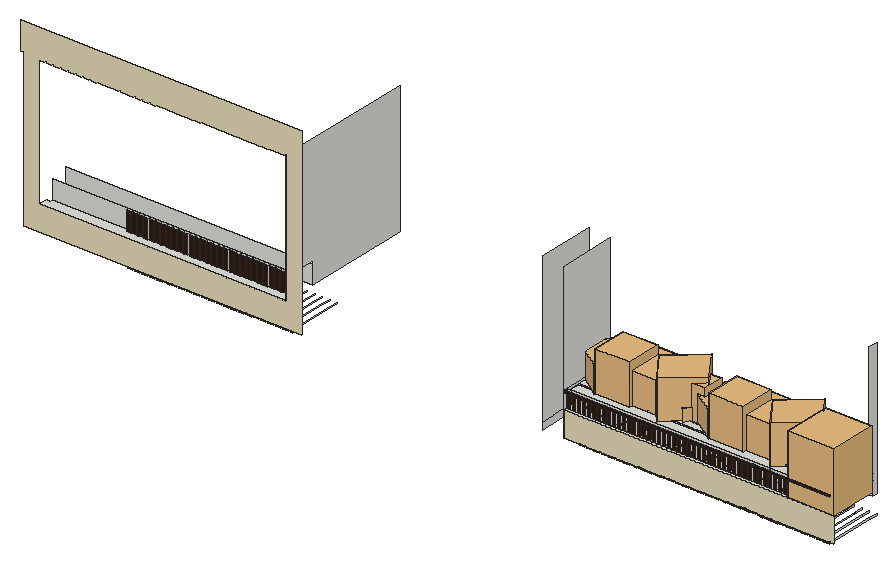
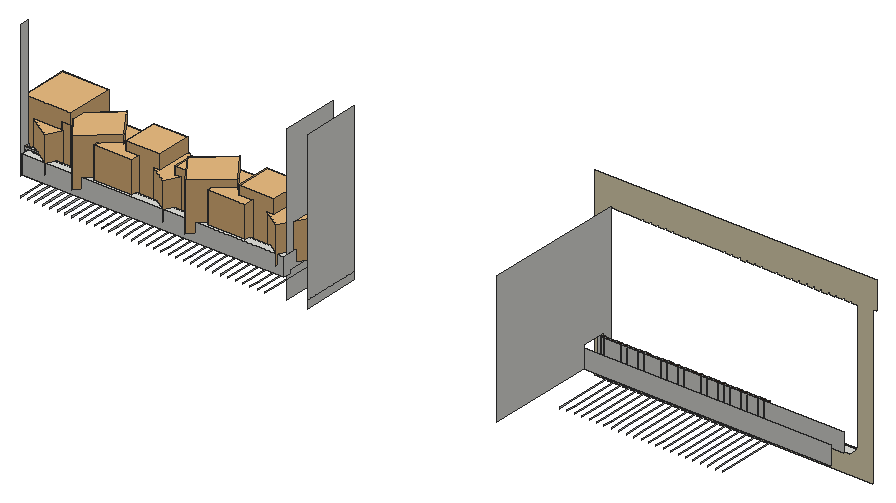
# SketchUp Ruby script. Lengths in inches.
U = 1.inch
M = Sketchup.active_model
def pt(a) = Geom::Point3d.new(a.map { |v| v * U })
def face(e, loops, mat)
  f = e.add_face(loops[0].map { |a| pt(a) })
  loops[1..].each { |l| e.add_face(l.map { |a| pt(a) }).erase! }
  f.material = f.back_material = mat if mat
  f
end
# faces: each face lists its corners as indices into pts; further lists are holes
def faces(e, pts, list, mat = nil) = list.each { |f| face(e, (f[0].is_a?(Array) ? f : [f]).map { |l| l.map { |i| pts[i] } }, mat) }
# xy, xz, yz: faces in a plane at the given z, y or x. An outline is a flat list of corners, or four numbers for a rectangle; further outlines are holes
def ring(l) = l.size == 4 ? [[l[0], l[1]], [l[2], l[1]], [l[2], l[3]], [l[0], l[3]]] : l.each_slice(2).to_a
def flat(e, list, mat, &to3) = list.each { |f| face(e, (f[0].is_a?(Array) ? f : [f]).map { |l| ring(l).map { |u, v| to3.(u, v) } }, mat) }
def xy(e, z, list, mat = nil) = flat(e, list, mat) { |x, y| [x, y, z] }
def xz(e, y, list, mat = nil) = flat(e, list, mat) { |x, z| [x, y, z] }
def yz(e, x, list, mat = nil) = flat(e, list, mat) { |y, z| [x, y, z] }
def lines(e, pts, list) = list.each { |a, b| e.add_line(pt(pts[a]), pt(pts[b])) }
# prism: a flat outline (further loops are holes) pulled along v
def prism(e, loops, v, mat = nil)
  f = face(e, loops, mat); d = Geom::Vector3d.new(v.map { |x| x * U })
  f.pushpull(f.normal.samedirection?(d) ? d.length : -d.length)
end
def box(e, o, s, mat = nil) = prism(e, [[o, [o[0] + s[0], o[1], o[2]], [o[0] + s[0], o[1] + s[1], o[2]], [o[0], o[1] + s[1], o[2]]]], [0, 0, s[2]], mat)
def at(x, y, z, deg = 0) = Geom::Transformation.translation(pt([x, y, z])) * Geom::Transformation.rotation(ORIGIN, Z_AXIS, deg.degrees)
def axes(o, x, y, z) = Geom::Transformation.new([*x, 0, *y, 0, *z, 0, *pt(o).to_a, 1])
def part(name) = M.definitions.add(name)
# library, detail: a bought-in or finely detailed component or shape, given as its bounding box
def library(name, o, s) = part(name).tap { |d| box(d.entities, o, s) }
def detail(e, o, s) = box(e.add_group.entities, o, s)
def put(e, d, t, mat = nil) = e.add_instance(d, t).tap { |i| i.material = mat if mat }
def group(e, t, mat = nil) = e.add_group.tap { |g| g.transformation = t; g.material = mat if mat }.entities
root = M.entities
M.materials.add("Material__1").color = [95, 70, 46]
M.materials.add("[Color D01]").color = [237, 225, 189]
M.materials.add("[Wood Veneer 01]").color = [51, 28, 15]
c1 = library("Areca palm plant",[0,0,0],[49.1,36.6,54.46])
c2 = library("Group\#74",[-84.69,-90.07,-0.36],[176.51,175.13,171.4])
c3 = library("Group20\#1",[-20.81,-17.08,3.79],[39.86,39.43,37.51])
c4 = library("Group\#130",[-7.34,-1.2,0],[38.67,35.81,49.04])
c5 = library("Group38\#2",[14.01,28.44,-23.43],[18.58,18.32,38.89])
c6 = part("Group\#16")
put(c6.entities,c1,axes([-6.2,158.41,6.08],[0.45017,-0.56191,0],[0.66137,0.52986,0],[0,0,0.72]))
put(c6.entities,c1,axes([-6.2,56.6,6.08],[0.45017,-0.56191,0],[0.66137,0.52986,0],[0,0,0.72]))
put(c6.entities,c2,axes([14.93,145.87,6.05],[-0.04961,-0.08593,0],[0.08593,-0.04961,0],[0,0,0.10522]))
put(c6.entities,c3,axes([18.97,79.98,4.77],[0,0.85,0],[-0.85,0,0],[0,0,0.85]))
put(c6.entities,c2,axes([14.93,173.12,6.05],[-0.04961,-0.08593,0],[0.08593,-0.04961,0],[0,0,0.10522]))
put(c6.entities,c2,axes([14.93,193.18,6.05],[-0.04961,-0.08593,0],[0.08593,-0.04961,0],[0,0,0.10522]))
put(c6.entities,c4,axes([24.9375,89.91,8],[0,0.79,0],[-0.79,0,0],[0,0,0.79]))
put(c6.entities,c5,axes([-4.1,-1.15,28.17],[0.8848,0,0],[0,0.94674,0],[0,0,0.85826]))
g1 = group(c6.entities,at(0,0,0))
xy(g1,0,[[0,0,6,234.8],[30,0,36,234.8]])
xy(g1,3,[[6,0,30,234.8]])
xy(g1,7,[[6,5,30,229.8]],"Material__1")
xy(g1,15,[[[0,0,36,234.8],[6,5,30,229.8]]])
xz(g1,0,[[0,0,6,0,6,3,30,3,30,0,36,0,36,15,0,15]])
xz(g1,5,[[6,7,30,15]])
xz(g1,229.8,[[6,7,30,15]])
xz(g1,234.8,[[0,0,0,15,36,15,36,0,30,0,30,3,6,3,6,0]])
yz(g1,0,[[0,0,234.8,15]])
yz(g1,6,[[0,0,234.8,3],[5,7,229.8,15]])
yz(g1,30,[[0,0,234.8,3],[5,7,229.8,15]])
yz(g1,36,[[0,0,234.8,15]])
put(c6.entities,c2,axes([14.93,91.37,6.05],[-0.04961,-0.08593,0],[0.08593,-0.04961,0],[0,0,0.10522]))
put(c6.entities,c2,axes([14.93,44.05,6.05],[-0.04961,-0.08593,0],[0.08593,-0.04961,0],[0,0,0.10522]))
put(c6.entities,c4,axes([24.9375,191.72,8],[0,0.79,0],[-0.79,0,0],[0,0,0.79]))
put(c6.entities,c5,axes([-4.1,100.66,28.17],[0.8848,0,0],[0,0.94674,0],[0,0,0.85826]))
put(c6.entities,c2,axes([17.19,15.79,6.07],[-0.08133,-0.14087,0],[0.14087,-0.08133,0],[0,0,0.1725]))
put(c6.entities,c2,axes([14.93,71.3,6.05],[-0.04961,-0.08593,0],[0.08593,-0.04961,0],[0,0,0.10522]))
put(c6.entities,c2,axes([17.19,121.23,6.07],[-0.08133,-0.14087,0],[0.14087,-0.08133,0],[0,0,0.1725]))
put(c6.entities,c2,axes([17.19,223.04,6.07],[-0.08133,-0.14087,0],[0.14087,-0.08133,0],[0,0,0.1725]))
put(c6.entities,c3,axes([18.97,181.79,4.77],[0,0.85,0],[-0.85,0,0],[0,0,0.85]))
c7 = library("plant (1)",[-35.72,-28.42,0],[66.31,67.39,84.38])
xy(root,269.0625,[[833.74,253.58,833.74,271.8,1035.46,271.8,1035.46,290.02,1042.55,290.02,1042.55,253.58]])
xy(root,275.125,[[409.32,246.64,609.07,246.64,609.07,255.84,413.01,255.84,413.01,253.84,409.32,253.84],[833.74,246.64,1052.37,249.27],[833.74,249.27,1049,253.58],[1042.55,253.58,1049,290.02]])
xy(root,287.25,[[833.74,246.64,1049,249.27],[833.74,249.27,833.74,271.8,1035.46,271.8,1035.46,290.02,1049,290.02,1049,249.27]])
xz(root,246.64,[[978.25,254.625,983,254.6875]])
xz(root,246.64,[[[396.57,254.6875,622,254.6875,622,403.1875,393.95,403.1875,393.95,380.6875,396.57,380.6875],[409.32,275.125,409.32,379.5625,413.74,379.5625,413.74,380.6875,415.32,380.6875,415.32,379.5625,419.74,379.5625,419.74,380.6875,421.32,380.6875,421.32,379.5625,425.74,379.5625,425.74,380.6875,427.32,380.6875,427.32,379.5625,431.74,379.5625,431.74,380.6875,433.32,380.6875,433.32,379.5625,437.74,379.5625,437.74,380.6875,439.32,380.6875,439.32,379.5625,443.74,379.5625,443.74,380.6875,445.32,380.6875,445.32,379.5625,449.74,379.5625,449.74,380.6875,451.32,380.6875,451.32,379.5625,455.74,379.5625,455.74,380.6875,457.32,380.6875,457.32,379.5625,461.74,379.5625,461.74,380.6875,463.32,380.6875,463.32,379.5625,467.74,379.5625,467.74,380.6875,469.32,380.6875,469.32,379.5625,473.74,379.5625,473.74,380.6875,475.32,380.6875,475.32,379.5625,479.74,379.5625,479.74,380.6875,481.32,380.6875,481.32,379.5625,485.74,379.5625,485.74,380.6875,487.32,380.6875,487.32,379.5625,491.74,379.5625,491.74,380.6875,493.32,380.6875,493.32,379.5625,497.74,379.5625,497.74,380.6875,499.32,380.6875,499.32,379.5625,503.74,379.5625,503.74,380.6875,505.32,380.6875,505.32,380.0625,509.74,380.0625,509.74,380.6875,511.32,380.6875,511.32,380.0625,515.74,380.0625,515.74,380.6875,517.32,380.6875,517.32,380.0625,521.74,380.0625,521.74,380.6875,523.32,380.6875,523.32,380.0625,527.74,380.0625,527.74,380.6875,529.32,380.6875,529.32,380.0625,533.74,380.0625,533.74,380.6875,535.32,380.6875,535.32,380.0625,539.74,380.0625,539.74,380.6875,541.32,380.6875,541.32,380.0625,545.74,380.0625,545.74,380.6875,547.32,380.6875,547.32,380.0625,551.74,380.0625,551.74,380.6875,553.32,380.6875,553.32,380.0625,557.74,380.0625,557.74,380.6875,559.32,380.6875,559.32,380.0625,563.74,380.0625,563.74,380.6875,565.32,380.6875,565.32,380.0625,569.74,380.0625,569.74,380.6875,571.32,380.6875,571.32,380.1875,575.74,380.1875,575.74,380.6875,577.32,380.6875,577.32,380.1875,581.74,380.1875,581.74,380.6875,583.32,380.6875,583.32,380.1875,587.74,380.1875,587.74,380.6875,589.32,380.6875,589.32,380.1875,593.74,380.1875,593.74,380.6875,595.32,380.6875,595.32,380.1875,599.74,380.1875,599.74,380.6875,601.32,380.6875,601.32,380.1875,605.74,380.1875,605.74,380.6875,609.07,380.6875,609.07,275.125]],[833.74,254.6875,1052.37,275.125]],"[Color D01]")
xz(root,246.64,[[990.25,253.5625,995,254.6875],[996.25,253.5625,1001,254.6875],[1002.25,253.5625,1007,254.6875],[1008.25,253.5625,1013,254.6875],[1014.25,253.5625,1019,254.6875],
  [1020.25,253.5625,1025,254.6875],[1026.25,253.5625,1031,254.6875],[1032.25,253.5625,1037,254.6875],[1038.25,253.5625,1043,254.6875],[1044.25,253.5625,1049,254.6875],
  [978.25,253.875,983,254.625],[984.25,253.875,989,254.6875],[480.57,253.9375,484.96,254.6875],[486.57,253.9375,490.96,254.6875],[492.57,253.9375,496.96,254.6875],
  [498.57,253.9375,502.96,254.6875],[504.57,253.9375,508.96,254.6875],[510.57,253.9375,514.96,254.6875],[516.57,253.9375,520.96,254.6875],[522.57,253.9375,526.96,254.6875],
  [528.57,253.9375,532.96,254.6875],[534.57,253.9375,538.96,254.6875],[540.57,253.9375,544.96,254.6875],[546.57,253.9375,550.96,254.6875],[552.57,253.9375,556.96,254.6875],
  [558.57,253.9375,562.96,254.6875],[564.57,253.9375,568.96,254.6875],[570.57,253.9375,574.96,254.6875],[576.57,253.9375,580.96,254.6875],[582.57,253.9375,586.96,254.6875],
  [588.57,253.9375,592.96,254.6875],[594.57,253.9375,598.96,254.6875],[600.57,253.9375,604.96,254.6875],[606.57,253.9375,610.96,254.6875],[612.57,253.9375,614.76,254.6875],
  [846.25,253.9375,851,254.6875],[852.25,253.9375,857,254.6875],[858.25,253.9375,863,254.6875],[864.25,253.9375,869,254.6875],[870.25,253.9375,875,254.6875],
  [876.25,253.9375,881,254.6875],[882.25,253.9375,887,254.6875],[888.25,253.9375,893,254.6875],[894.25,253.9375,899,254.6875],[900.25,253.9375,905,254.6875],
  [906.25,253.9375,911,254.6875],[912.25,253.9375,917,254.6875],[918.25,253.9375,923,254.6875],[924.25,253.9375,929,254.6875],[930.25,253.9375,935,254.6875],
  [936.25,253.9375,941,254.6875],[942.25,253.9375,947,254.6875],[948.25,253.9375,953,254.6875],[954.25,253.9375,959,254.6875],[960.25,253.9375,965,254.6875],
  [966.25,253.9375,971,254.6875],[972.25,253.9375,977,254.6875],[833.74,287.25,1049,289.1875]],"[Wood Veneer 01]")
xz(root,249.27,[[837.02,275.125,837.8,287.25],[841.08,275.125,841.86,287.25],[845.14,275.125,845.93,287.25],[849.2,275.125,849.99,287.25],[853.27,275.125,854.05,287.25],
  [857.33,275.125,858.11,287.25],[861.39,275.125,862.18,287.25],[865.45,275.125,866.24,287.25],[869.52,275.125,870.3,287.25],[873.58,275.125,874.36,287.25],
  [877.64,275.125,878.43,287.25],[881.7,275.125,882.49,287.25],[885.77,275.125,886.55,287.25],[889.83,275.125,890.61,287.25],[893.89,275.125,894.68,287.25],
  [897.95,275.125,898.74,287.25],[902.02,275.125,902.8,287.25],[906.08,275.125,906.86,287.25],[910.14,275.125,910.93,287.25],[914.2,275.125,914.99,287.25],
  [918.27,275.125,919.05,287.25],[922.33,275.125,923.11,287.25],[926.39,275.125,927.18,287.25],[930.45,275.125,931.24,287.25],[934.52,275.125,935.3,287.25],
  [938.58,275.125,939.36,287.25],[942.64,275.125,943.43,287.25],[946.7,275.125,947.49,287.25],[950.77,275.125,951.55,287.25],[954.83,275.125,955.61,287.25],
  [958.89,275.125,959.68,287.25],[962.95,275.125,963.74,287.25],[967.02,275.125,967.8,287.25],[971.08,275.125,971.86,287.25],[975.14,275.125,975.93,287.25],
  [979.2,275.125,979.99,287.25],[983.27,275.125,984.05,287.25],[987.33,275.125,988.11,287.25],[991.39,275.125,992.18,287.25],[995.45,275.125,996.24,287.25],
  [999.52,275.125,1000.3,287.25],[1003.58,275.125,1004.36,287.25],[1007.64,275.125,1008.43,287.25],[1011.7,275.125,1012.49,287.25],[1015.77,275.125,1016.55,287.25],
  [1019.83,275.125,1020.61,287.25],[1023.89,275.125,1024.68,287.25],[1027.95,275.125,1028.74,287.25],[1032.02,275.125,1032.8,287.25],[1036.08,275.125,1036.86,287.25],
  [1040.14,275.125,1040.93,287.25],[1044.2,275.125,1044.99,287.25],[1048.27,275.125,1049,287.25],[833.74,287.25,837.02,289.1875],[837.02,287.25,1049,289.1875]])
xz(root,249.27,[[833.74,275.125,837.02,287.25],[837.8,275.125,841.08,287.25],[841.86,275.125,845.14,287.25],[845.93,275.125,849.2,287.25],[849.99,275.125,853.27,287.25],
  [854.05,275.125,857.33,287.25],[858.11,275.125,861.39,287.25],[862.18,275.125,865.45,287.25],[866.24,275.125,869.52,287.25],[870.3,275.125,873.58,287.25],
  [874.36,275.125,877.64,287.25],[878.43,275.125,881.7,287.25],[882.49,275.125,885.77,287.25],[886.55,275.125,889.83,287.25],[890.61,275.125,893.89,287.25],
  [894.68,275.125,897.95,287.25],[898.74,275.125,902.02,287.25],[902.8,275.125,906.08,287.25],[906.86,275.125,910.14,287.25],[910.93,275.125,914.2,287.25],
  [914.99,275.125,918.27,287.25],[919.05,275.125,922.33,287.25],[923.11,275.125,926.39,287.25],[927.18,275.125,930.45,287.25],[931.24,275.125,934.52,287.25],
  [935.3,275.125,938.58,287.25],[939.36,275.125,942.64,287.25],[943.43,275.125,946.7,287.25],[947.49,275.125,950.77,287.25],[951.55,275.125,954.83,287.25],
  [955.61,275.125,958.89,287.25],[959.68,275.125,962.95,287.25],[963.74,275.125,967.02,287.25],[967.8,275.125,971.08,287.25],[971.86,275.125,975.14,287.25],
  [975.93,275.125,979.2,287.25],[979.99,275.125,983.27,287.25],[984.05,275.125,987.33,287.25],[988.11,275.125,991.39,287.25],[992.18,275.125,995.45,287.25],
  [996.24,275.125,999.52,287.25],[1000.3,275.125,1003.58,287.25],[1004.36,275.125,1007.64,287.25],[1008.43,275.125,1011.7,287.25],[1012.49,275.125,1015.77,287.25],
  [1016.55,275.125,1019.83,287.25],[1020.61,275.125,1023.89,287.25],[1024.68,275.125,1027.95,287.25],[1028.74,275.125,1032.02,287.25],[1032.8,275.125,1036.08,287.25],
  [1036.86,275.125,1040.14,287.25],[1040.93,275.125,1044.2,287.25],[1044.99,275.125,1048.27,287.25]],"[Wood Veneer 01]")
xz(root,253.58,[[833.74,269.0625,1042.55,275.125]])
xz(root,253.84,[[474.07,275.125,477.76,290.375],[478.7,275.125,482.39,290.375],[483.32,275.125,487.01,290.375],[487.95,275.125,491.64,290.375],[492.57,275.125,496.26,290.375],
  [497.2,275.125,500.89,290.375],[501.82,275.125,505.51,290.375],[506.45,275.125,510.14,290.375],[511.07,275.125,514.76,290.375],[515.7,275.125,519.39,290.375],
  [520.32,275.125,524.01,290.375],[524.95,275.125,528.64,290.375],[529.57,275.125,533.26,290.375],[534.2,275.125,537.89,290.375],[538.82,275.125,542.51,290.375],
  [543.45,275.125,547.14,290.375],[548.07,275.125,551.76,290.375],[552.7,275.125,556.39,290.375],[557.32,275.125,561.01,290.375],[561.95,275.125,565.64,290.375],
  [566.57,275.125,570.26,290.375],[571.2,275.125,574.89,290.375],[575.82,275.125,579.51,290.375],[580.45,275.125,584.14,290.375],[585.07,275.125,588.76,290.375],
  [589.7,275.125,593.39,290.375],[594.32,275.125,598.01,290.375],[598.95,275.125,602.64,290.375],[603.57,275.125,607.26,290.375],[608.2,275.125,611.89,290.375]],"[Wood Veneer 01]")
xz(root,255.84,[[413.01,275.125,609.07,290.375]])
xz(root,271.8,[[833.74,269.0625,1035.46,287.25],[833.74,287.25,1035.46,289.1875]])
xz(root,273.33,[[409.32,275.125,609.07,290.375]])
xz(root,290.02,[[1035.46,269.0625,1035.46,287.25,1049,287.25,1049,275.125,1042.55,275.125,1042.55,269.0625],[1042.55,269.0625,1049,275.125],[1035.46,287.25,1049,289.1875]])
yz(root,477.76,[[253.84,275.125,255.47,290.375]])
yz(root,480.57,[[246.64,253.9375,286.21,254.6875],[286.21,253.9375,293.45,254.6875]])
yz(root,482.39,[[253.84,275.125,255.47,290.375]])
yz(root,486.57,[[246.64,253.9375,286.21,254.6875],[286.21,253.9375,293.45,254.6875]])
yz(root,487.01,[[253.84,275.125,255.47,290.375]])
yz(root,491.64,[[253.84,275.125,255.47,290.375]])
yz(root,492.57,[[246.64,253.9375,286.21,254.6875],[286.21,253.9375,293.45,254.6875]])
yz(root,496.26,[[253.84,275.125,255.47,290.375]])
yz(root,498.57,[[246.64,253.9375,286.21,254.6875],[286.21,253.9375,293.45,254.6875]])
yz(root,500.89,[[253.84,275.125,255.47,290.375]])
yz(root,504.57,[[246.64,253.9375,286.21,254.6875],[286.21,253.9375,293.45,254.6875]])
yz(root,505.51,[[253.84,275.125,255.47,290.375]])
yz(root,510.14,[[253.84,275.125,255.47,290.375]])
yz(root,510.57,[[246.64,253.9375,286.21,254.6875],[286.21,253.9375,293.45,254.6875]])
yz(root,514.76,[[253.84,275.125,255.47,290.375]])
yz(root,516.57,[[246.64,253.9375,286.21,254.6875],[286.21,253.9375,293.45,254.6875]])
yz(root,519.39,[[253.84,275.125,255.47,290.375]])
yz(root,522.57,[[246.64,253.9375,286.21,254.6875],[286.21,253.9375,293.45,254.6875]])
yz(root,524.01,[[253.84,275.125,255.47,290.375]])
yz(root,528.57,[[246.64,253.9375,286.21,254.6875],[286.21,253.9375,293.45,254.6875]])
yz(root,528.64,[[253.84,275.125,255.47,290.375]])
yz(root,533.26,[[253.84,275.125,255.47,290.375]])
yz(root,534.57,[[246.64,253.9375,286.21,254.6875],[286.21,253.9375,293.45,254.6875]])
yz(root,537.89,[[253.84,275.125,255.47,290.375]])
yz(root,540.57,[[246.64,253.9375,286.21,254.6875],[286.21,253.9375,293.45,254.6875]])
yz(root,542.51,[[253.84,275.125,255.47,290.375]])
yz(root,546.57,[[246.64,253.9375,286.21,254.6875],[286.21,253.9375,293.45,254.6875]])
yz(root,547.14,[[253.84,275.125,255.47,290.375]])
yz(root,551.76,[[253.84,275.125,255.47,290.375]])
yz(root,552.57,[[246.64,253.9375,286.21,254.6875],[286.21,253.9375,293.45,254.6875]])
yz(root,556.39,[[253.84,275.125,255.47,290.375]])
yz(root,558.57,[[246.64,253.9375,286.21,254.6875],[286.21,253.9375,293.45,254.6875]])
yz(root,561.01,[[253.84,275.125,255.47,290.375]])
yz(root,564.57,[[246.64,253.9375,286.21,254.6875],[286.21,253.9375,293.45,254.6875]])
yz(root,565.64,[[253.84,275.125,255.47,290.375]])
yz(root,570.26,[[253.84,275.125,255.47,290.375]])
yz(root,570.57,[[246.64,253.9375,286.21,254.6875],[286.21,253.9375,293.45,254.6875]])
yz(root,574.89,[[253.84,275.125,255.47,290.375]])
yz(root,576.57,[[246.64,253.9375,286.21,254.6875],[286.21,253.9375,293.45,254.6875]])
yz(root,579.51,[[253.84,275.125,255.47,290.375]])
yz(root,582.57,[[246.64,253.9375,286.21,254.6875],[286.21,253.9375,293.45,254.6875]])
yz(root,584.14,[[253.84,275.125,255.47,290.375]])
yz(root,588.57,[[246.64,253.9375,286.21,254.6875],[286.21,253.9375,293.45,254.6875]])
yz(root,588.76,[[253.84,275.125,255.47,290.375]])
yz(root,593.39,[[253.84,275.125,255.47,290.375]])
yz(root,594.57,[[246.64,253.9375,286.21,254.6875],[286.21,253.9375,293.45,254.6875]])
yz(root,598.01,[[253.84,275.125,255.47,290.375]])
yz(root,600.57,[[246.64,253.9375,286.21,254.6875],[286.21,253.9375,293.45,254.6875]])
yz(root,602.64,[[253.84,275.125,255.47,290.375]])
yz(root,606.57,[[246.64,253.9375,286.21,254.6875],[286.21,253.9375,293.45,254.6875]])
yz(root,607.26,[[253.84,275.125,255.47,290.375]])
yz(root,609.07,[[246.64,275.125,246.64,380.6875,361.27,380.6875,361.27,275.125,273.33,275.125,273.33,292.5625,253.22,292.5625,253.22,290.375,255.84,290.375,255.84,275.125]])
yz(root,611.89,[[253.84,275.125,255.47,290.375]])
yz(root,612.57,[[246.64,253.9375,286.21,254.6875],[286.21,253.9375,293.45,254.6875]])
yz(root,816.6875,[[246.64,254.6875,293.46,260.6875],[246.64,260.6875,293.46,380.6875]])
yz(root,833.74,[[246.64,254.6875,293.46,254.6875,293.46,269.0625,253.58,269.0625,253.58,275.125,246.64,275.125],[253.58,269.0625,271.8,275.125],[271.8,269.0625,293.46,275.125],[246.64,275.125,249.27,287.25],[271.8,275.125,293.46,275.125,293.46,378.875,246.64,378.875,246.64,289.1875,271.8,289.1875],
  [249.27,275.125,271.8,287.25],[246.64,287.25,249.27,289.1875],[249.27,287.25,271.8,289.1875]])
yz(root,851,[[246.64,253.9375,286.21,254.6875],[286.21,253.9375,293.45,254.6875]])
yz(root,857,[[246.64,253.9375,286.21,254.6875],[286.21,253.9375,293.45,254.6875]])
yz(root,863,[[246.64,253.9375,286.21,254.6875],[286.21,253.9375,293.45,254.6875]])
yz(root,869,[[246.64,253.9375,286.21,254.6875],[286.21,253.9375,293.45,254.6875]])
yz(root,875,[[246.64,253.9375,286.21,254.6875],[286.21,253.9375,293.45,254.6875]])
yz(root,881,[[246.64,253.9375,286.21,254.6875],[286.21,253.9375,293.45,254.6875]])
yz(root,887,[[246.64,253.9375,286.21,254.6875],[286.21,253.9375,293.45,254.6875]])
yz(root,893,[[246.64,253.9375,286.21,254.6875],[286.21,253.9375,293.45,254.6875]])
yz(root,899,[[246.64,253.9375,286.21,254.6875],[286.21,253.9375,293.45,254.6875]])
yz(root,905,[[246.64,253.9375,286.21,254.6875],[286.21,253.9375,293.45,254.6875]])
yz(root,911,[[246.64,253.9375,286.21,254.6875],[286.21,253.9375,293.45,254.6875]])
yz(root,917,[[246.64,253.9375,286.21,254.6875],[286.21,253.9375,293.45,254.6875]])
yz(root,923,[[246.64,253.9375,286.21,254.6875],[286.21,253.9375,293.45,254.6875]])
yz(root,929,[[246.64,253.9375,286.21,254.6875],[286.21,253.9375,293.45,254.6875]])
yz(root,935,[[246.64,253.9375,286.21,254.6875],[286.21,253.9375,293.45,254.6875]])
yz(root,941,[[246.64,253.9375,286.21,254.6875],[286.21,253.9375,293.45,254.6875]])
yz(root,947,[[246.64,253.9375,286.21,254.6875],[286.21,253.9375,293.45,254.6875]])
yz(root,953,[[246.64,253.9375,286.21,254.6875],[286.21,253.9375,293.45,254.6875]])
yz(root,959,[[246.64,253.9375,286.21,254.6875],[286.21,253.9375,293.45,254.6875]])
yz(root,965,[[246.64,253.9375,286.21,254.6875],[286.21,253.9375,293.45,254.6875]])
yz(root,971,[[246.64,253.9375,286.21,254.6875],[286.21,253.9375,293.45,254.6875]])
yz(root,977,[[246.64,253.9375,286.21,254.6875],[286.21,253.9375,293.45,254.6875]])
yz(root,983,[[246.64,253.875,286.21,254.625],[286.21,253.875,293.45,254.625],[246.64,254.625,286.21,254.6875],[286.21,254.625,293.45,254.6875]])
yz(root,989,[[246.64,253.875,286.21,254.6875],[286.21,253.875,293.45,254.6875]])
yz(root,995,[[246.64,253.5625,286.21,254.6875],[286.21,253.5625,293.45,254.6875]])
yz(root,1001,[[246.64,253.5625,286.21,254.6875],[286.21,253.5625,293.45,254.6875]])
yz(root,1007,[[246.64,253.5625,286.21,254.6875],[286.21,253.5625,293.45,254.6875]])
yz(root,1013,[[246.64,253.5625,286.21,254.6875],[286.21,253.5625,293.45,254.6875]])
yz(root,1019,[[246.64,253.5625,286.21,254.6875],[286.21,253.5625,293.45,254.6875]])
yz(root,1025,[[246.64,253.5625,286.21,254.6875],[286.21,253.5625,293.45,254.6875]])
yz(root,1031,[[246.64,253.5625,286.21,254.6875],[286.21,253.5625,293.45,254.6875]])
yz(root,1035.46,[[271.8,269.0625,290.02,287.25],[271.8,287.25,290.02,289.1875]])
yz(root,1037,[[246.64,253.5625,286.21,254.6875],[286.21,253.5625,293.45,254.6875]])
yz(root,1042.55,[[253.58,269.0625,290.02,275.125]])
yz(root,1043,[[246.64,253.5625,286.21,254.6875],[286.21,253.5625,293.45,254.6875]])
yz(root,1049,[[246.64,253.5625,286.21,254.6875],[286.21,253.5625,293.45,254.6875],[290.02,269.0625,290.02,289.1875,286.21,289.1875,286.21,378.875,293.45,378.875,293.45,269.0625],[249.27,275.125,286.21,287.25],[286.21,275.125,290.02,287.25],
  [249.27,287.25,286.21,289.1875]])
put(root,c6,axes([1045.33,260.97,273.05],[0,1,0],[-0.9045,0,0],[0,0,1]))
put(root,c7,axes([1034.9375,262.85,275.125],[0.57,0,0],[0,0.57,0],[0,0,0.57]))
